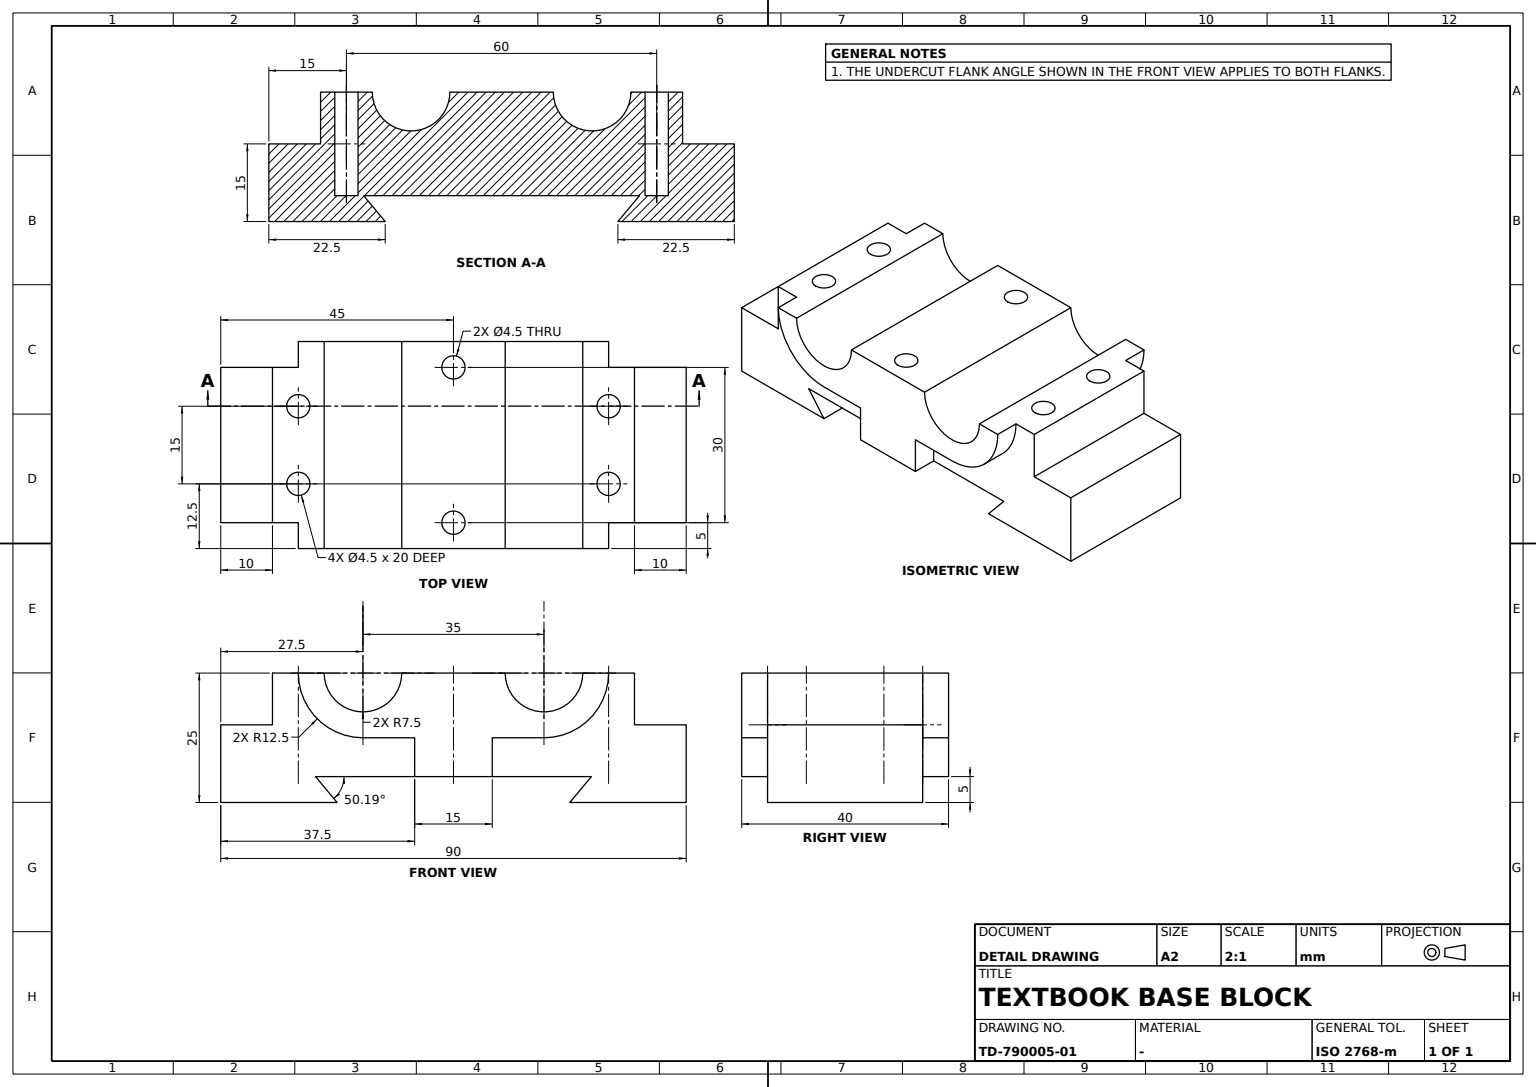
ISO-10303-21;
HEADER;
FILE_DESCRIPTION((''),'2;1');
FILE_NAME('','',(''),(''),'','','');
FILE_SCHEMA(('AUTOMOTIVE_DESIGN'));
ENDSEC;
DATA;
#1=APPLICATION_CONTEXT('');
#2=PRODUCT_CONTEXT('',#1,'mechanical');
#3=PRODUCT('','','',(#2));
#4=PRODUCT_DEFINITION_FORMATION('','',#3);
#5=PRODUCT_DEFINITION_CONTEXT('',#1,'design');
#6=PRODUCT_DEFINITION('','',#4,#5);
#7=PRODUCT_DEFINITION_SHAPE('','',#6);
#8=(LENGTH_UNIT()NAMED_UNIT(*)SI_UNIT(.MILLI.,.METRE.));
#9=(NAMED_UNIT(*)PLANE_ANGLE_UNIT()SI_UNIT($,.RADIAN.));
#10=(NAMED_UNIT(*)SI_UNIT($,.STERADIAN.)SOLID_ANGLE_UNIT());
#11=UNCERTAINTY_MEASURE_WITH_UNIT(LENGTH_MEASURE(0.005),#8,'distance_accuracy_value','');
#12=(GEOMETRIC_REPRESENTATION_CONTEXT(3)GLOBAL_UNCERTAINTY_ASSIGNED_CONTEXT((#11))GLOBAL_UNIT_ASSIGNED_CONTEXT((#8,#9,#10))REPRESENTATION_CONTEXT('',''));
#13=CARTESIAN_POINT('',(15.,35.,20.));
#14=VERTEX_POINT('',#13);
#15=CARTESIAN_POINT('',(15.,30.,20.));
#16=VERTEX_POINT('',#15);
#17=CARTESIAN_POINT('',(15.,0.,20.));
#18=DIRECTION('',(0.,-1.,0.));
#19=VECTOR('',#18,1000.);
#20=LINE('',#17,#19);
#21=EDGE_CURVE('',#14,#16,#20,.T.);
#22=ORIENTED_EDGE('',*,*,#21,.F.);
#23=CARTESIAN_POINT('',(-15.,35.,20.));
#24=VERTEX_POINT('',#23);
#25=CARTESIAN_POINT('',(0.,35.,20.));
#26=DIRECTION('',(1.,0.,0.));
#27=VECTOR('',#26,1000.);
#28=LINE('',#25,#27);
#29=EDGE_CURVE('',#24,#14,#28,.T.);
#30=ORIENTED_EDGE('',*,*,#29,.F.);
#31=CARTESIAN_POINT('',(-15.,30.,20.));
#32=VERTEX_POINT('',#31);
#33=CARTESIAN_POINT('',(-15.,0.,20.));
#34=LINE('',#33,#19);
#35=EDGE_CURVE('',#24,#32,#34,.T.);
#36=ORIENTED_EDGE('',*,*,#35,.T.);
#37=CARTESIAN_POINT('',(-20.,30.,20.));
#38=VERTEX_POINT('',#37);
#39=LINE('',#31,#27);
#40=EDGE_CURVE('',#32,#38,#39,.F.);
#41=ORIENTED_EDGE('',*,*,#40,.T.);
#42=CARTESIAN_POINT('',(-20.,25.,20.));
#43=VERTEX_POINT('',#42);
#44=CARTESIAN_POINT('',(-20.,0.,20.));
#45=LINE('',#44,#19);
#46=EDGE_CURVE('',#38,#43,#45,.T.);
#47=ORIENTED_EDGE('',*,*,#46,.T.);
#48=CARTESIAN_POINT('',(20.,25.,20.));
#49=VERTEX_POINT('',#48);
#50=LINE('',#42,#27);
#51=EDGE_CURVE('',#43,#49,#50,.T.);
#52=ORIENTED_EDGE('',*,*,#51,.T.);
#53=CARTESIAN_POINT('',(20.,30.,20.));
#54=VERTEX_POINT('',#53);
#55=CARTESIAN_POINT('',(20.,0.,20.));
#56=LINE('',#55,#19);
#57=EDGE_CURVE('',#54,#49,#56,.T.);
#58=ORIENTED_EDGE('',*,*,#57,.F.);
#59=LINE('',#15,#27);
#60=EDGE_CURVE('',#16,#54,#59,.T.);
#61=ORIENTED_EDGE('',*,*,#60,.F.);
#62=EDGE_LOOP('',(#22,#30,#36,#41,#47,#52,#58,#61));
#63=FACE_BOUND('',#62,.T.);
#64=CARTESIAN_POINT('',(9.75,30.,20.));
#65=VERTEX_POINT('',#64);
#66=CARTESIAN_POINT('',(7.5,30.,20.));
#67=DIRECTION('',(0.,0.,1.));
#68=AXIS2_PLACEMENT_3D('',#66,#67,#26);
#69=CIRCLE('',#68,2.25);
#70=EDGE_CURVE('',#65,#65,#69,.T.);
#71=ORIENTED_EDGE('',*,*,#70,.F.);
#72=EDGE_LOOP('',(#71));
#73=FACE_BOUND('',#72,.T.);
#74=CARTESIAN_POINT('',(-5.25,30.,20.));
#75=VERTEX_POINT('',#74);
#76=CARTESIAN_POINT('',(-7.5,30.,20.));
#77=AXIS2_PLACEMENT_3D('',#76,#67,#26);
#78=CIRCLE('',#77,2.25);
#79=EDGE_CURVE('',#75,#75,#78,.T.);
#80=ORIENTED_EDGE('',*,*,#79,.F.);
#81=EDGE_LOOP('',(#80));
#82=FACE_BOUND('',#81,.T.);
#83=AXIS2_PLACEMENT_3D('',#25,#67,#18);
#84=PLANE('',#83);
#85=ADVANCED_FACE('',(#63,#73,#82),#84,.T.);
#86=CARTESIAN_POINT('',(-9.75,-30.,0.));
#87=VERTEX_POINT('',#86);
#88=CARTESIAN_POINT('',(-7.5,-30.,0.));
#89=DIRECTION('',(0.,0.,-1.));
#90=DIRECTION('',(-1.,0.,0.));
#91=AXIS2_PLACEMENT_3D('',#88,#89,#90);
#92=CIRCLE('',#91,2.25);
#93=EDGE_CURVE('',#87,#87,#92,.F.);
#94=ORIENTED_EDGE('',*,*,#93,.T.);
#95=EDGE_LOOP('',(#94));
#96=FACE_BOUND('',#95,.T.);
#97=CARTESIAN_POINT('',(0.,-26.666667,0.));
#98=DIRECTION('',(0.,1.,0.));
#99=AXIS2_PLACEMENT_3D('',#97,#89,#98);
#100=PLANE('',#99);
#101=ADVANCED_FACE('',(#96),#100,.F.);
#102=CARTESIAN_POINT('',(-15.,-35.,10.));
#103=VERTEX_POINT('',#102);
#104=CARTESIAN_POINT('',(15.,-35.,10.));
#105=VERTEX_POINT('',#104);
#106=CARTESIAN_POINT('',(0.,-35.,10.));
#107=LINE('',#106,#27);
#108=EDGE_CURVE('',#103,#105,#107,.T.);
#109=ORIENTED_EDGE('',*,*,#108,.F.);
#110=CARTESIAN_POINT('',(-15.,-45.,10.));
#111=VERTEX_POINT('',#110);
#112=CARTESIAN_POINT('',(-15.,45.,10.));
#113=VECTOR('',#98,1000.);
#114=LINE('',#112,#113);
#115=EDGE_CURVE('',#111,#103,#114,.T.);
#116=ORIENTED_EDGE('',*,*,#115,.F.);
#117=CARTESIAN_POINT('',(15.,-45.,10.));
#118=VERTEX_POINT('',#117);
#119=CARTESIAN_POINT('',(0.,-45.,10.));
#120=LINE('',#119,#27);
#121=EDGE_CURVE('',#111,#118,#120,.T.);
#122=ORIENTED_EDGE('',*,*,#121,.T.);
#123=CARTESIAN_POINT('',(15.,45.,10.));
#124=LINE('',#123,#113);
#125=EDGE_CURVE('',#118,#105,#124,.T.);
#126=ORIENTED_EDGE('',*,*,#125,.T.);
#127=EDGE_LOOP('',(#109,#116,#122,#126));
#128=FACE_BOUND('',#127,.T.);
#129=CARTESIAN_POINT('',(0.,45.,10.));
#130=AXIS2_PLACEMENT_3D('',#129,#67,#18);
#131=PLANE('',#130);
#132=ADVANCED_FACE('',(#128),#131,.T.);
#133=CARTESIAN_POINT('',(-15.,35.,10.));
#134=VERTEX_POINT('',#133);
#135=CARTESIAN_POINT('',(15.,35.,10.));
#136=VERTEX_POINT('',#135);
#137=CARTESIAN_POINT('',(0.,35.,10.));
#138=LINE('',#137,#27);
#139=EDGE_CURVE('',#134,#136,#138,.T.);
#140=ORIENTED_EDGE('',*,*,#139,.F.);
#141=CARTESIAN_POINT('',(-15.,35.,0.));
#142=VECTOR('',#67,1000.);
#143=LINE('',#141,#142);
#144=EDGE_CURVE('',#134,#24,#143,.T.);
#145=ORIENTED_EDGE('',*,*,#144,.T.);
#146=ORIENTED_EDGE('',*,*,#29,.T.);
#147=CARTESIAN_POINT('',(15.,35.,0.));
#148=LINE('',#147,#142);
#149=EDGE_CURVE('',#136,#14,#148,.T.);
#150=ORIENTED_EDGE('',*,*,#149,.F.);
#151=EDGE_LOOP('',(#140,#145,#146,#150));
#152=FACE_BOUND('',#151,.T.);
#153=AXIS2_PLACEMENT_3D('',#137,#98,#67);
#154=PLANE('',#153);
#155=ADVANCED_FACE('',(#152),#154,.T.);
#156=CARTESIAN_POINT('',(12.75,0.,0.));
#157=VERTEX_POINT('',#156);
#158=CARTESIAN_POINT('',(15.,0.,0.));
#159=AXIS2_PLACEMENT_3D('',#158,#89,#90);
#160=CIRCLE('',#159,2.25);
#161=EDGE_CURVE('',#157,#157,#160,.F.);
#162=ORIENTED_EDGE('',*,*,#161,.F.);
#163=EDGE_LOOP('',(#162));
#164=FACE_BOUND('',#163,.T.);
#165=CARTESIAN_POINT('',(17.25,0.,20.));
#166=VERTEX_POINT('',#165);
#167=AXIS2_PLACEMENT_3D('',#17,#67,#26);
#168=CIRCLE('',#167,2.25);
#169=EDGE_CURVE('',#166,#166,#168,.T.);
#170=ORIENTED_EDGE('',*,*,#169,.T.);
#171=EDGE_LOOP('',(#170));
#172=FACE_BOUND('',#171,.T.);
#173=CARTESIAN_POINT('',(15.,0.,10.66));
#174=AXIS2_PLACEMENT_3D('',#173,#67,#26);
#175=CYLINDRICAL_SURFACE('',#174,2.25);
#176=ADVANCED_FACE('',(#164,#172),#175,.F.);
#177=CARTESIAN_POINT('',(-15.,-17.5,7.5));
#178=VERTEX_POINT('',#177);
#179=CARTESIAN_POINT('',(-15.,-7.5,7.5));
#180=VERTEX_POINT('',#179);
#181=CARTESIAN_POINT('',(-15.,0.,7.5));
#182=LINE('',#181,#113);
#183=EDGE_CURVE('',#178,#180,#182,.T.);
#184=ORIENTED_EDGE('',*,*,#183,.F.);
#185=CARTESIAN_POINT('',(-20.,-17.5,7.5));
#186=VERTEX_POINT('',#185);
#187=CARTESIAN_POINT('',(17.5,-17.5,7.5));
#188=LINE('',#187,#27);
#189=EDGE_CURVE('',#178,#186,#188,.F.);
#190=ORIENTED_EDGE('',*,*,#189,.T.);
#191=CARTESIAN_POINT('',(-20.,-7.5,7.5));
#192=VERTEX_POINT('',#191);
#193=CARTESIAN_POINT('',(-20.,0.,7.5));
#194=LINE('',#193,#113);
#195=EDGE_CURVE('',#186,#192,#194,.T.);
#196=ORIENTED_EDGE('',*,*,#195,.T.);
#197=CARTESIAN_POINT('',(15.,-7.5,7.5));
#198=VECTOR('',#90,1000.);
#199=LINE('',#197,#198);
#200=EDGE_CURVE('',#180,#192,#199,.T.);
#201=ORIENTED_EDGE('',*,*,#200,.F.);
#202=EDGE_LOOP('',(#184,#190,#196,#201));
#203=FACE_BOUND('',#202,.T.);
#204=CARTESIAN_POINT('',(15.,-17.5,7.5));
#205=AXIS2_PLACEMENT_3D('',#204,#89,#98);
#206=PLANE('',#205);
#207=ADVANCED_FACE('',(#203),#206,.T.);
#208=CARTESIAN_POINT('',(15.,-45.,-5.));
#209=VERTEX_POINT('',#208);
#210=CARTESIAN_POINT('',(15.,-45.,0.));
#211=LINE('',#210,#142);
#212=EDGE_CURVE('',#209,#118,#211,.T.);
#213=ORIENTED_EDGE('',*,*,#212,.T.);
#214=ORIENTED_EDGE('',*,*,#121,.F.);
#215=CARTESIAN_POINT('',(-15.,-45.,-5.));
#216=VERTEX_POINT('',#215);
#217=CARTESIAN_POINT('',(-15.,-45.,0.));
#218=LINE('',#217,#142);
#219=EDGE_CURVE('',#216,#111,#218,.T.);
#220=ORIENTED_EDGE('',*,*,#219,.F.);
#221=CARTESIAN_POINT('',(0.,-45.,-5.));
#222=LINE('',#221,#27);
#223=EDGE_CURVE('',#216,#209,#222,.T.);
#224=ORIENTED_EDGE('',*,*,#223,.T.);
#225=EDGE_LOOP('',(#213,#214,#220,#224));
#226=FACE_BOUND('',#225,.T.);
#227=AXIS2_PLACEMENT_3D('',#221,#98,#67);
#228=PLANE('',#227);
#229=ADVANCED_FACE('',(#226),#228,.F.);
#230=CARTESIAN_POINT('',(15.,45.,-5.));
#231=VERTEX_POINT('',#230);
#232=VERTEX_POINT('',#123);
#233=CARTESIAN_POINT('',(15.,45.,0.));
#234=LINE('',#233,#142);
#235=EDGE_CURVE('',#231,#232,#234,.T.);
#236=ORIENTED_EDGE('',*,*,#235,.F.);
#237=CARTESIAN_POINT('',(-15.,45.,-5.));
#238=VERTEX_POINT('',#237);
#239=CARTESIAN_POINT('',(0.,45.,-5.));
#240=LINE('',#239,#27);
#241=EDGE_CURVE('',#238,#231,#240,.T.);
#242=ORIENTED_EDGE('',*,*,#241,.F.);
#243=VERTEX_POINT('',#112);
#244=CARTESIAN_POINT('',(-15.,45.,0.));
#245=LINE('',#244,#142);
#246=EDGE_CURVE('',#238,#243,#245,.T.);
#247=ORIENTED_EDGE('',*,*,#246,.T.);
#248=LINE('',#129,#27);
#249=EDGE_CURVE('',#243,#232,#248,.T.);
#250=ORIENTED_EDGE('',*,*,#249,.T.);
#251=EDGE_LOOP('',(#236,#242,#247,#250));
#252=FACE_BOUND('',#251,.T.);
#253=AXIS2_PLACEMENT_3D('',#239,#98,#67);
#254=PLANE('',#253);
#255=ADVANCED_FACE('',(#252),#254,.T.);
#256=CARTESIAN_POINT('',(-20.,-7.5,0.));
#257=VERTEX_POINT('',#256);
#258=CARTESIAN_POINT('',(-20.,7.5,0.));
#259=VERTEX_POINT('',#258);
#260=CARTESIAN_POINT('',(-20.,0.,0.));
#261=LINE('',#260,#113);
#262=EDGE_CURVE('',#257,#259,#261,.T.);
#263=ORIENTED_EDGE('',*,*,#262,.F.);
#264=VECTOR('',#89,1000.);
#265=LINE('',#256,#264);
#266=EDGE_CURVE('',#192,#257,#265,.T.);
#267=ORIENTED_EDGE('',*,*,#266,.F.);
#268=ORIENTED_EDGE('',*,*,#195,.F.);
#269=CARTESIAN_POINT('',(-20.,-30.,20.));
#270=VERTEX_POINT('',#269);
#271=CARTESIAN_POINT('',(-20.,-17.5,20.));
#272=AXIS2_PLACEMENT_3D('',#271,#26,#89);
#273=CIRCLE('',#272,12.5);
#274=EDGE_CURVE('',#270,#186,#273,.T.);
#275=ORIENTED_EDGE('',*,*,#274,.F.);
#276=CARTESIAN_POINT('',(-20.,-25.,20.));
#277=VERTEX_POINT('',#276);
#278=CARTESIAN_POINT('',(-20.,35.,20.));
#279=LINE('',#278,#113);
#280=EDGE_CURVE('',#270,#277,#279,.T.);
#281=ORIENTED_EDGE('',*,*,#280,.T.);
#282=CARTESIAN_POINT('',(-20.,-10.,20.));
#283=VERTEX_POINT('',#282);
#284=CIRCLE('',#272,7.5);
#285=EDGE_CURVE('',#277,#283,#284,.T.);
#286=ORIENTED_EDGE('',*,*,#285,.T.);
#287=CARTESIAN_POINT('',(-20.,10.,20.));
#288=VERTEX_POINT('',#287);
#289=EDGE_CURVE('',#288,#283,#45,.T.);
#290=ORIENTED_EDGE('',*,*,#289,.F.);
#291=CARTESIAN_POINT('',(-20.,17.5,20.));
#292=AXIS2_PLACEMENT_3D('',#291,#26,#89);
#293=CIRCLE('',#292,7.5);
#294=EDGE_CURVE('',#288,#43,#293,.T.);
#295=ORIENTED_EDGE('',*,*,#294,.T.);
#296=ORIENTED_EDGE('',*,*,#46,.F.);
#297=CARTESIAN_POINT('',(-20.,17.5,7.5));
#298=VERTEX_POINT('',#297);
#299=CIRCLE('',#292,12.5);
#300=EDGE_CURVE('',#298,#38,#299,.T.);
#301=ORIENTED_EDGE('',*,*,#300,.F.);
#302=CARTESIAN_POINT('',(-20.,7.5,7.5));
#303=VERTEX_POINT('',#302);
#304=LINE('',#185,#19);
#305=EDGE_CURVE('',#298,#303,#304,.T.);
#306=ORIENTED_EDGE('',*,*,#305,.T.);
#307=LINE('',#258,#264);
#308=EDGE_CURVE('',#303,#259,#307,.T.);
#309=ORIENTED_EDGE('',*,*,#308,.T.);
#310=EDGE_LOOP('',(#263,#267,#268,#275,#281,#286,#290,#295,#296,#301,#306,#309));
#311=FACE_BOUND('',#310,.T.);
#312=AXIS2_PLACEMENT_3D('',#260,#26,#98);
#313=PLANE('',#312);
#314=ADVANCED_FACE('',(#311),#313,.F.);
#315=CARTESIAN_POINT('',(5.25,-30.,0.));
#316=VERTEX_POINT('',#315);
#317=CARTESIAN_POINT('',(7.5,-30.,0.));
#318=AXIS2_PLACEMENT_3D('',#317,#89,#90);
#319=CIRCLE('',#318,2.25);
#320=EDGE_CURVE('',#316,#316,#319,.F.);
#321=ORIENTED_EDGE('',*,*,#320,.T.);
#322=EDGE_LOOP('',(#321));
#323=FACE_BOUND('',#322,.T.);
#324=ADVANCED_FACE('',(#323),#100,.F.);
#325=CARTESIAN_POINT('',(-15.,22.5,-5.));
#326=VERTEX_POINT('',#325);
#327=CARTESIAN_POINT('',(15.,22.5,-5.));
#328=VERTEX_POINT('',#327);
#329=CARTESIAN_POINT('',(0.,22.5,-5.));
#330=LINE('',#329,#27);
#331=EDGE_CURVE('',#326,#328,#330,.T.);
#332=ORIENTED_EDGE('',*,*,#331,.T.);
#333=CARTESIAN_POINT('',(15.,26.666667,0.));
#334=VERTEX_POINT('',#333);
#335=CARTESIAN_POINT('',(15.,15.737705,-13.114754));
#336=DIRECTION('',(0.,0.6401844,0.76822128));
#337=VECTOR('',#336,1000.);
#338=LINE('',#335,#337);
#339=EDGE_CURVE('',#328,#334,#338,.T.);
#340=ORIENTED_EDGE('',*,*,#339,.T.);
#341=CARTESIAN_POINT('',(-15.,26.666667,0.));
#342=VERTEX_POINT('',#341);
#343=CARTESIAN_POINT('',(0.,26.666667,0.));
#344=LINE('',#343,#27);
#345=EDGE_CURVE('',#342,#334,#344,.T.);
#346=ORIENTED_EDGE('',*,*,#345,.F.);
#347=CARTESIAN_POINT('',(-15.,15.737705,-13.114754));
#348=LINE('',#347,#337);
#349=EDGE_CURVE('',#326,#342,#348,.T.);
#350=ORIENTED_EDGE('',*,*,#349,.F.);
#351=EDGE_LOOP('',(#332,#340,#346,#350));
#352=FACE_BOUND('',#351,.T.);
#353=DIRECTION('',(0.,0.76822128,-0.6401844));
#354=AXIS2_PLACEMENT_3D('',#329,#353,#336);
#355=PLANE('',#354);
#356=ADVANCED_FACE('',(#352),#355,.F.);
#357=CARTESIAN_POINT('',(5.25,30.,0.));
#358=VERTEX_POINT('',#357);
#359=CARTESIAN_POINT('',(7.5,30.,0.));
#360=AXIS2_PLACEMENT_3D('',#359,#89,#90);
#361=CIRCLE('',#360,2.25);
#362=EDGE_CURVE('',#358,#358,#361,.F.);
#363=ORIENTED_EDGE('',*,*,#362,.T.);
#364=EDGE_LOOP('',(#363));
#365=FACE_BOUND('',#364,.T.);
#366=ADVANCED_FACE('',(#365),#100,.F.);
#367=ORIENTED_EDGE('',*,*,#223,.F.);
#368=CARTESIAN_POINT('',(-15.,-22.5,-5.));
#369=VERTEX_POINT('',#368);
#370=CARTESIAN_POINT('',(-15.,0.,-5.));
#371=LINE('',#370,#113);
#372=EDGE_CURVE('',#216,#369,#371,.T.);
#373=ORIENTED_EDGE('',*,*,#372,.T.);
#374=CARTESIAN_POINT('',(15.,-22.5,-5.));
#375=VERTEX_POINT('',#374);
#376=CARTESIAN_POINT('',(0.,-22.5,-5.));
#377=LINE('',#376,#27);
#378=EDGE_CURVE('',#369,#375,#377,.T.);
#379=ORIENTED_EDGE('',*,*,#378,.T.);
#380=CARTESIAN_POINT('',(15.,0.,-5.));
#381=LINE('',#380,#113);
#382=EDGE_CURVE('',#209,#375,#381,.T.);
#383=ORIENTED_EDGE('',*,*,#382,.F.);
#384=EDGE_LOOP('',(#367,#373,#379,#383));
#385=FACE_BOUND('',#384,.T.);
#386=AXIS2_PLACEMENT_3D('',#221,#89,#98);
#387=PLANE('',#386);
#388=ADVANCED_FACE('',(#385),#387,.T.);
#389=CARTESIAN_POINT('',(9.75,-30.,20.));
#390=VERTEX_POINT('',#389);
#391=CARTESIAN_POINT('',(7.5,-30.,20.));
#392=AXIS2_PLACEMENT_3D('',#391,#67,#26);
#393=CIRCLE('',#392,2.25);
#394=EDGE_CURVE('',#390,#390,#393,.T.);
#395=ORIENTED_EDGE('',*,*,#394,.T.);
#396=EDGE_LOOP('',(#395));
#397=FACE_BOUND('',#396,.T.);
#398=ORIENTED_EDGE('',*,*,#320,.F.);
#399=EDGE_LOOP('',(#398));
#400=FACE_BOUND('',#399,.T.);
#401=CARTESIAN_POINT('',(7.5,-30.,10.66));
#402=AXIS2_PLACEMENT_3D('',#401,#67,#26);
#403=CYLINDRICAL_SURFACE('',#402,2.25);
#404=ADVANCED_FACE('',(#397,#400),#403,.F.);
#405=ORIENTED_EDGE('',*,*,#382,.T.);
#406=CARTESIAN_POINT('',(15.,-26.666667,0.));
#407=VERTEX_POINT('',#406);
#408=CARTESIAN_POINT('',(15.,-15.737705,-13.114754));
#409=DIRECTION('',(0.,-0.6401844,0.76822128));
#410=VECTOR('',#409,1000.);
#411=LINE('',#408,#410);
#412=EDGE_CURVE('',#375,#407,#411,.T.);
#413=ORIENTED_EDGE('',*,*,#412,.T.);
#414=CARTESIAN_POINT('',(15.,-7.5,0.));
#415=VERTEX_POINT('',#414);
#416=LINE('',#158,#113);
#417=EDGE_CURVE('',#407,#415,#416,.T.);
#418=ORIENTED_EDGE('',*,*,#417,.T.);
#419=VERTEX_POINT('',#197);
#420=LINE('',#414,#264);
#421=EDGE_CURVE('',#419,#415,#420,.T.);
#422=ORIENTED_EDGE('',*,*,#421,.F.);
#423=VERTEX_POINT('',#204);
#424=CARTESIAN_POINT('',(15.,0.,7.5));
#425=LINE('',#424,#113);
#426=EDGE_CURVE('',#423,#419,#425,.T.);
#427=ORIENTED_EDGE('',*,*,#426,.F.);
#428=CARTESIAN_POINT('',(15.,-30.,20.));
#429=VERTEX_POINT('',#428);
#430=CARTESIAN_POINT('',(15.,-17.5,20.));
#431=AXIS2_PLACEMENT_3D('',#430,#26,#89);
#432=CIRCLE('',#431,12.5);
#433=EDGE_CURVE('',#429,#423,#432,.T.);
#434=ORIENTED_EDGE('',*,*,#433,.F.);
#435=CARTESIAN_POINT('',(15.,-35.,20.));
#436=VERTEX_POINT('',#435);
#437=LINE('',#13,#113);
#438=EDGE_CURVE('',#436,#429,#437,.T.);
#439=ORIENTED_EDGE('',*,*,#438,.F.);
#440=CARTESIAN_POINT('',(15.,-35.,0.));
#441=LINE('',#440,#142);
#442=EDGE_CURVE('',#105,#436,#441,.T.);
#443=ORIENTED_EDGE('',*,*,#442,.F.);
#444=ORIENTED_EDGE('',*,*,#125,.F.);
#445=ORIENTED_EDGE('',*,*,#212,.F.);
#446=EDGE_LOOP('',(#405,#413,#418,#422,#427,#434,#439,#443,#444,#445));
#447=FACE_BOUND('',#446,.T.);
#448=AXIS2_PLACEMENT_3D('',#158,#26,#98);
#449=PLANE('',#448);
#450=ADVANCED_FACE('',(#447),#449,.T.);
#451=ORIENTED_EDGE('',*,*,#339,.F.);
#452=LINE('',#208,#19);
#453=EDGE_CURVE('',#231,#328,#452,.T.);
#454=ORIENTED_EDGE('',*,*,#453,.F.);
#455=ORIENTED_EDGE('',*,*,#235,.T.);
#456=CARTESIAN_POINT('',(15.,0.,10.));
#457=LINE('',#456,#19);
#458=EDGE_CURVE('',#232,#136,#457,.T.);
#459=ORIENTED_EDGE('',*,*,#458,.T.);
#460=ORIENTED_EDGE('',*,*,#149,.T.);
#461=ORIENTED_EDGE('',*,*,#21,.T.);
#462=CARTESIAN_POINT('',(15.,17.5,7.5));
#463=VERTEX_POINT('',#462);
#464=CARTESIAN_POINT('',(15.,17.5,20.));
#465=AXIS2_PLACEMENT_3D('',#464,#26,#89);
#466=CIRCLE('',#465,12.5);
#467=EDGE_CURVE('',#463,#16,#466,.T.);
#468=ORIENTED_EDGE('',*,*,#467,.F.);
#469=CARTESIAN_POINT('',(15.,7.5,7.5));
#470=VERTEX_POINT('',#469);
#471=LINE('',#204,#19);
#472=EDGE_CURVE('',#463,#470,#471,.T.);
#473=ORIENTED_EDGE('',*,*,#472,.T.);
#474=CARTESIAN_POINT('',(15.,7.5,0.));
#475=VERTEX_POINT('',#474);
#476=LINE('',#474,#264);
#477=EDGE_CURVE('',#470,#475,#476,.T.);
#478=ORIENTED_EDGE('',*,*,#477,.T.);
#479=EDGE_CURVE('',#475,#334,#416,.T.);
#480=ORIENTED_EDGE('',*,*,#479,.T.);
#481=EDGE_LOOP('',(#451,#454,#455,#459,#460,#461,#468,#473,#478,#480));
#482=FACE_BOUND('',#481,.T.);
#483=ADVANCED_FACE('',(#482),#449,.T.);
#484=ORIENTED_EDGE('',*,*,#274,.T.);
#485=ORIENTED_EDGE('',*,*,#189,.F.);
#486=CARTESIAN_POINT('',(-15.,-30.,20.));
#487=VERTEX_POINT('',#486);
#488=CARTESIAN_POINT('',(-15.,-17.5,20.));
#489=AXIS2_PLACEMENT_3D('',#488,#26,#89);
#490=CIRCLE('',#489,12.5);
#491=EDGE_CURVE('',#487,#178,#490,.T.);
#492=ORIENTED_EDGE('',*,*,#491,.F.);
#493=LINE('',#486,#27);
#494=EDGE_CURVE('',#487,#270,#493,.F.);
#495=ORIENTED_EDGE('',*,*,#494,.T.);
#496=EDGE_LOOP('',(#484,#485,#492,#495));
#497=FACE_BOUND('',#496,.T.);
#498=CARTESIAN_POINT('',(17.5,-17.5,20.));
#499=AXIS2_PLACEMENT_3D('',#498,#26,#98);
#500=CYLINDRICAL_SURFACE('',#499,12.5);
#501=ADVANCED_FACE('',(#497),#500,.T.);
#502=ORIENTED_EDGE('',*,*,#169,.F.);
#503=EDGE_LOOP('',(#502));
#504=FACE_BOUND('',#503,.T.);
#505=CARTESIAN_POINT('',(20.,-10.,20.));
#506=VERTEX_POINT('',#505);
#507=LINE('',#282,#27);
#508=EDGE_CURVE('',#283,#506,#507,.T.);
#509=ORIENTED_EDGE('',*,*,#508,.T.);
#510=CARTESIAN_POINT('',(20.,10.,20.));
#511=VERTEX_POINT('',#510);
#512=EDGE_CURVE('',#511,#506,#56,.T.);
#513=ORIENTED_EDGE('',*,*,#512,.F.);
#514=LINE('',#287,#27);
#515=EDGE_CURVE('',#288,#511,#514,.T.);
#516=ORIENTED_EDGE('',*,*,#515,.F.);
#517=ORIENTED_EDGE('',*,*,#289,.T.);
#518=EDGE_LOOP('',(#509,#513,#516,#517));
#519=FACE_BOUND('',#518,.T.);
#520=CARTESIAN_POINT('',(-12.75,0.,20.));
#521=VERTEX_POINT('',#520);
#522=AXIS2_PLACEMENT_3D('',#33,#67,#26);
#523=CIRCLE('',#522,2.25);
#524=EDGE_CURVE('',#521,#521,#523,.T.);
#525=ORIENTED_EDGE('',*,*,#524,.F.);
#526=EDGE_LOOP('',(#525));
#527=FACE_BOUND('',#526,.T.);
#528=ADVANCED_FACE('',(#504,#519,#527),#84,.T.);
#529=CARTESIAN_POINT('',(-5.25,-30.,20.));
#530=VERTEX_POINT('',#529);
#531=CARTESIAN_POINT('',(-7.5,-30.,20.));
#532=AXIS2_PLACEMENT_3D('',#531,#67,#26);
#533=CIRCLE('',#532,2.25);
#534=EDGE_CURVE('',#530,#530,#533,.T.);
#535=ORIENTED_EDGE('',*,*,#534,.F.);
#536=EDGE_LOOP('',(#535));
#537=FACE_BOUND('',#536,.T.);
#538=ORIENTED_EDGE('',*,*,#394,.F.);
#539=EDGE_LOOP('',(#538));
#540=FACE_BOUND('',#539,.T.);
#541=CARTESIAN_POINT('',(-15.,-35.,20.));
#542=VERTEX_POINT('',#541);
#543=LINE('',#23,#113);
#544=EDGE_CURVE('',#542,#487,#543,.T.);
#545=ORIENTED_EDGE('',*,*,#544,.F.);
#546=CARTESIAN_POINT('',(0.,-35.,20.));
#547=LINE('',#546,#27);
#548=EDGE_CURVE('',#542,#436,#547,.T.);
#549=ORIENTED_EDGE('',*,*,#548,.T.);
#550=ORIENTED_EDGE('',*,*,#438,.T.);
#551=CARTESIAN_POINT('',(20.,-30.,20.));
#552=VERTEX_POINT('',#551);
#553=LINE('',#428,#27);
#554=EDGE_CURVE('',#429,#552,#553,.T.);
#555=ORIENTED_EDGE('',*,*,#554,.T.);
#556=CARTESIAN_POINT('',(20.,-25.,20.));
#557=VERTEX_POINT('',#556);
#558=CARTESIAN_POINT('',(20.,35.,20.));
#559=LINE('',#558,#113);
#560=EDGE_CURVE('',#552,#557,#559,.T.);
#561=ORIENTED_EDGE('',*,*,#560,.T.);
#562=LINE('',#276,#27);
#563=EDGE_CURVE('',#277,#557,#562,.T.);
#564=ORIENTED_EDGE('',*,*,#563,.F.);
#565=ORIENTED_EDGE('',*,*,#280,.F.);
#566=ORIENTED_EDGE('',*,*,#494,.F.);
#567=EDGE_LOOP('',(#545,#549,#550,#555,#561,#564,#565,#566));
#568=FACE_BOUND('',#567,.T.);
#569=ADVANCED_FACE('',(#537,#540,#568),#84,.T.);
#570=CARTESIAN_POINT('',(-15.,17.5,7.5));
#571=VERTEX_POINT('',#570);
#572=CARTESIAN_POINT('',(-15.,17.5,20.));
#573=AXIS2_PLACEMENT_3D('',#572,#26,#89);
#574=CIRCLE('',#573,12.5);
#575=EDGE_CURVE('',#571,#32,#574,.T.);
#576=ORIENTED_EDGE('',*,*,#575,.F.);
#577=CARTESIAN_POINT('',(17.5,17.5,7.5));
#578=LINE('',#577,#27);
#579=EDGE_CURVE('',#571,#298,#578,.F.);
#580=ORIENTED_EDGE('',*,*,#579,.T.);
#581=ORIENTED_EDGE('',*,*,#300,.T.);
#582=ORIENTED_EDGE('',*,*,#40,.F.);
#583=EDGE_LOOP('',(#576,#580,#581,#582));
#584=FACE_BOUND('',#583,.T.);
#585=CARTESIAN_POINT('',(17.5,17.5,20.));
#586=AXIS2_PLACEMENT_3D('',#585,#26,#98);
#587=CYLINDRICAL_SURFACE('',#586,12.5);
#588=ADVANCED_FACE('',(#584),#587,.T.);
#589=ORIENTED_EDGE('',*,*,#241,.T.);
#590=ORIENTED_EDGE('',*,*,#453,.T.);
#591=ORIENTED_EDGE('',*,*,#331,.F.);
#592=LINE('',#215,#19);
#593=EDGE_CURVE('',#238,#326,#592,.T.);
#594=ORIENTED_EDGE('',*,*,#593,.F.);
#595=EDGE_LOOP('',(#589,#590,#591,#594));
#596=FACE_BOUND('',#595,.T.);
#597=ADVANCED_FACE('',(#596),#387,.T.);
#598=CARTESIAN_POINT('',(20.,7.5,7.5));
#599=VERTEX_POINT('',#598);
#600=LINE('',#469,#27);
#601=EDGE_CURVE('',#470,#599,#600,.T.);
#602=ORIENTED_EDGE('',*,*,#601,.F.);
#603=ORIENTED_EDGE('',*,*,#472,.F.);
#604=CARTESIAN_POINT('',(20.,17.5,7.5));
#605=VERTEX_POINT('',#604);
#606=EDGE_CURVE('',#463,#605,#578,.T.);
#607=ORIENTED_EDGE('',*,*,#606,.T.);
#608=CARTESIAN_POINT('',(20.,-17.5,7.5));
#609=LINE('',#608,#19);
#610=EDGE_CURVE('',#605,#599,#609,.T.);
#611=ORIENTED_EDGE('',*,*,#610,.T.);
#612=EDGE_LOOP('',(#602,#603,#607,#611));
#613=FACE_BOUND('',#612,.T.);
#614=ADVANCED_FACE('',(#613),#206,.T.);
#615=ORIENTED_EDGE('',*,*,#308,.F.);
#616=CARTESIAN_POINT('',(-15.,7.5,7.5));
#617=VERTEX_POINT('',#616);
#618=LINE('',#469,#198);
#619=EDGE_CURVE('',#617,#303,#618,.T.);
#620=ORIENTED_EDGE('',*,*,#619,.F.);
#621=CARTESIAN_POINT('',(-15.,7.5,0.));
#622=VERTEX_POINT('',#621);
#623=LINE('',#621,#264);
#624=EDGE_CURVE('',#617,#622,#623,.T.);
#625=ORIENTED_EDGE('',*,*,#624,.T.);
#626=CARTESIAN_POINT('',(0.,7.5,0.));
#627=LINE('',#626,#198);
#628=EDGE_CURVE('',#622,#259,#627,.T.);
#629=ORIENTED_EDGE('',*,*,#628,.T.);
#630=EDGE_LOOP('',(#615,#620,#625,#629));
#631=FACE_BOUND('',#630,.T.);
#632=AXIS2_PLACEMENT_3D('',#469,#18,#89);
#633=PLANE('',#632);
#634=ADVANCED_FACE('',(#631),#633,.F.);
#635=ORIENTED_EDGE('',*,*,#285,.F.);
#636=ORIENTED_EDGE('',*,*,#563,.T.);
#637=CARTESIAN_POINT('',(20.,-17.5,20.));
#638=AXIS2_PLACEMENT_3D('',#637,#26,#89);
#639=CIRCLE('',#638,7.5);
#640=EDGE_CURVE('',#557,#506,#639,.T.);
#641=ORIENTED_EDGE('',*,*,#640,.T.);
#642=ORIENTED_EDGE('',*,*,#508,.F.);
#643=EDGE_LOOP('',(#635,#636,#641,#642));
#644=FACE_BOUND('',#643,.T.);
#645=CARTESIAN_POINT('',(0.,-17.5,20.));
#646=AXIS2_PLACEMENT_3D('',#645,#26,#98);
#647=CYLINDRICAL_SURFACE('',#646,7.5);
#648=ADVANCED_FACE('',(#644),#647,.F.);
#649=CARTESIAN_POINT('',(-15.,0.,10.));
#650=LINE('',#649,#19);
#651=EDGE_CURVE('',#243,#134,#650,.T.);
#652=ORIENTED_EDGE('',*,*,#651,.F.);
#653=ORIENTED_EDGE('',*,*,#246,.F.);
#654=ORIENTED_EDGE('',*,*,#593,.T.);
#655=ORIENTED_EDGE('',*,*,#349,.T.);
#656=CARTESIAN_POINT('',(-15.,0.,0.));
#657=LINE('',#656,#113);
#658=EDGE_CURVE('',#622,#342,#657,.T.);
#659=ORIENTED_EDGE('',*,*,#658,.F.);
#660=ORIENTED_EDGE('',*,*,#624,.F.);
#661=LINE('',#177,#19);
#662=EDGE_CURVE('',#571,#617,#661,.T.);
#663=ORIENTED_EDGE('',*,*,#662,.F.);
#664=ORIENTED_EDGE('',*,*,#575,.T.);
#665=ORIENTED_EDGE('',*,*,#35,.F.);
#666=ORIENTED_EDGE('',*,*,#144,.F.);
#667=EDGE_LOOP('',(#652,#653,#654,#655,#659,#660,#663,#664,#665,#666));
#668=FACE_BOUND('',#667,.T.);
#669=AXIS2_PLACEMENT_3D('',#656,#26,#98);
#670=PLANE('',#669);
#671=ADVANCED_FACE('',(#668),#670,.F.);
#672=VERTEX_POINT('',#608);
#673=CIRCLE('',#638,12.5);
#674=EDGE_CURVE('',#552,#672,#673,.T.);
#675=ORIENTED_EDGE('',*,*,#674,.F.);
#676=ORIENTED_EDGE('',*,*,#554,.F.);
#677=ORIENTED_EDGE('',*,*,#433,.T.);
#678=EDGE_CURVE('',#423,#672,#188,.T.);
#679=ORIENTED_EDGE('',*,*,#678,.T.);
#680=EDGE_LOOP('',(#675,#676,#677,#679));
#681=FACE_BOUND('',#680,.T.);
#682=ADVANCED_FACE('',(#681),#500,.T.);
#683=ORIENTED_EDGE('',*,*,#601,.T.);
#684=CARTESIAN_POINT('',(20.,7.5,0.));
#685=VERTEX_POINT('',#684);
#686=LINE('',#684,#264);
#687=EDGE_CURVE('',#599,#685,#686,.T.);
#688=ORIENTED_EDGE('',*,*,#687,.T.);
#689=LINE('',#474,#27);
#690=EDGE_CURVE('',#475,#685,#689,.T.);
#691=ORIENTED_EDGE('',*,*,#690,.F.);
#692=ORIENTED_EDGE('',*,*,#477,.F.);
#693=EDGE_LOOP('',(#683,#688,#691,#692));
#694=FACE_BOUND('',#693,.T.);
#695=ADVANCED_FACE('',(#694),#633,.F.);
#696=ORIENTED_EDGE('',*,*,#515,.T.);
#697=CARTESIAN_POINT('',(20.,17.5,20.));
#698=AXIS2_PLACEMENT_3D('',#697,#26,#89);
#699=CIRCLE('',#698,7.5);
#700=EDGE_CURVE('',#511,#49,#699,.T.);
#701=ORIENTED_EDGE('',*,*,#700,.T.);
#702=ORIENTED_EDGE('',*,*,#51,.F.);
#703=ORIENTED_EDGE('',*,*,#294,.F.);
#704=EDGE_LOOP('',(#696,#701,#702,#703));
#705=FACE_BOUND('',#704,.T.);
#706=CARTESIAN_POINT('',(0.,17.5,20.));
#707=AXIS2_PLACEMENT_3D('',#706,#26,#98);
#708=CYLINDRICAL_SURFACE('',#707,7.5);
#709=ADVANCED_FACE('',(#705),#708,.F.);
#710=ORIENTED_EDGE('',*,*,#421,.T.);
#711=CARTESIAN_POINT('',(20.,-7.5,0.));
#712=VERTEX_POINT('',#711);
#713=LINE('',#414,#27);
#714=EDGE_CURVE('',#415,#712,#713,.T.);
#715=ORIENTED_EDGE('',*,*,#714,.T.);
#716=CARTESIAN_POINT('',(20.,-7.5,7.5));
#717=VERTEX_POINT('',#716);
#718=LINE('',#711,#264);
#719=EDGE_CURVE('',#717,#712,#718,.T.);
#720=ORIENTED_EDGE('',*,*,#719,.F.);
#721=LINE('',#197,#27);
#722=EDGE_CURVE('',#419,#717,#721,.T.);
#723=ORIENTED_EDGE('',*,*,#722,.F.);
#724=EDGE_LOOP('',(#710,#715,#720,#723));
#725=FACE_BOUND('',#724,.T.);
#726=AXIS2_PLACEMENT_3D('',#197,#18,#89);
#727=PLANE('',#726);
#728=ADVANCED_FACE('',(#725),#727,.T.);
#729=ORIENTED_EDGE('',*,*,#467,.T.);
#730=ORIENTED_EDGE('',*,*,#60,.T.);
#731=CIRCLE('',#698,12.5);
#732=EDGE_CURVE('',#605,#54,#731,.T.);
#733=ORIENTED_EDGE('',*,*,#732,.F.);
#734=ORIENTED_EDGE('',*,*,#606,.F.);
#735=EDGE_LOOP('',(#729,#730,#733,#734));
#736=FACE_BOUND('',#735,.T.);
#737=ADVANCED_FACE('',(#736),#587,.T.);
#738=CARTESIAN_POINT('',(-9.75,30.,0.));
#739=VERTEX_POINT('',#738);
#740=CARTESIAN_POINT('',(-7.5,30.,0.));
#741=AXIS2_PLACEMENT_3D('',#740,#89,#90);
#742=CIRCLE('',#741,2.25);
#743=EDGE_CURVE('',#739,#739,#742,.F.);
#744=ORIENTED_EDGE('',*,*,#743,.T.);
#745=EDGE_LOOP('',(#744));
#746=FACE_BOUND('',#745,.T.);
#747=ADVANCED_FACE('',(#746),#100,.F.);
#748=ORIENTED_EDGE('',*,*,#524,.T.);
#749=EDGE_LOOP('',(#748));
#750=FACE_BOUND('',#749,.T.);
#751=CARTESIAN_POINT('',(-17.25,0.,0.));
#752=VERTEX_POINT('',#751);
#753=AXIS2_PLACEMENT_3D('',#656,#89,#90);
#754=CIRCLE('',#753,2.25);
#755=EDGE_CURVE('',#752,#752,#754,.F.);
#756=ORIENTED_EDGE('',*,*,#755,.F.);
#757=EDGE_LOOP('',(#756));
#758=FACE_BOUND('',#757,.T.);
#759=CARTESIAN_POINT('',(-15.,0.,10.66));
#760=AXIS2_PLACEMENT_3D('',#759,#67,#26);
#761=CYLINDRICAL_SURFACE('',#760,2.25);
#762=ADVANCED_FACE('',(#750,#758),#761,.F.);
#763=ORIENTED_EDGE('',*,*,#619,.T.);
#764=ORIENTED_EDGE('',*,*,#305,.F.);
#765=ORIENTED_EDGE('',*,*,#579,.F.);
#766=ORIENTED_EDGE('',*,*,#662,.T.);
#767=EDGE_LOOP('',(#763,#764,#765,#766));
#768=FACE_BOUND('',#767,.T.);
#769=ADVANCED_FACE('',(#768),#206,.T.);
#770=ORIENTED_EDGE('',*,*,#442,.T.);
#771=ORIENTED_EDGE('',*,*,#548,.F.);
#772=CARTESIAN_POINT('',(-15.,-35.,0.));
#773=LINE('',#772,#142);
#774=EDGE_CURVE('',#103,#542,#773,.T.);
#775=ORIENTED_EDGE('',*,*,#774,.F.);
#776=ORIENTED_EDGE('',*,*,#108,.T.);
#777=EDGE_LOOP('',(#770,#771,#775,#776));
#778=FACE_BOUND('',#777,.T.);
#779=AXIS2_PLACEMENT_3D('',#106,#98,#67);
#780=PLANE('',#779);
#781=ADVANCED_FACE('',(#778),#780,.F.);
#782=CARTESIAN_POINT('',(-15.,-7.5,0.));
#783=VERTEX_POINT('',#782);
#784=CARTESIAN_POINT('',(0.,-7.5,0.));
#785=LINE('',#784,#198);
#786=EDGE_CURVE('',#783,#257,#785,.T.);
#787=ORIENTED_EDGE('',*,*,#786,.F.);
#788=LINE('',#782,#264);
#789=EDGE_CURVE('',#180,#783,#788,.T.);
#790=ORIENTED_EDGE('',*,*,#789,.F.);
#791=ORIENTED_EDGE('',*,*,#200,.T.);
#792=ORIENTED_EDGE('',*,*,#266,.T.);
#793=EDGE_LOOP('',(#787,#790,#791,#792));
#794=FACE_BOUND('',#793,.T.);
#795=ADVANCED_FACE('',(#794),#727,.T.);
#796=ORIENTED_EDGE('',*,*,#93,.F.);
#797=EDGE_LOOP('',(#796));
#798=FACE_BOUND('',#797,.T.);
#799=ORIENTED_EDGE('',*,*,#534,.T.);
#800=EDGE_LOOP('',(#799));
#801=FACE_BOUND('',#800,.T.);
#802=CARTESIAN_POINT('',(-7.5,-30.,10.66));
#803=AXIS2_PLACEMENT_3D('',#802,#67,#26);
#804=CYLINDRICAL_SURFACE('',#803,2.25);
#805=ADVANCED_FACE('',(#798,#801),#804,.F.);
#806=ORIENTED_EDGE('',*,*,#70,.T.);
#807=EDGE_LOOP('',(#806));
#808=FACE_BOUND('',#807,.T.);
#809=ORIENTED_EDGE('',*,*,#362,.F.);
#810=EDGE_LOOP('',(#809));
#811=FACE_BOUND('',#810,.T.);
#812=CARTESIAN_POINT('',(7.5,30.,10.66));
#813=AXIS2_PLACEMENT_3D('',#812,#67,#26);
#814=CYLINDRICAL_SURFACE('',#813,2.25);
#815=ADVANCED_FACE('',(#808,#811),#814,.F.);
#816=ORIENTED_EDGE('',*,*,#743,.F.);
#817=EDGE_LOOP('',(#816));
#818=FACE_BOUND('',#817,.T.);
#819=ORIENTED_EDGE('',*,*,#79,.T.);
#820=EDGE_LOOP('',(#819));
#821=FACE_BOUND('',#820,.T.);
#822=CARTESIAN_POINT('',(-7.5,30.,10.66));
#823=AXIS2_PLACEMENT_3D('',#822,#67,#26);
#824=CYLINDRICAL_SURFACE('',#823,2.25);
#825=ADVANCED_FACE('',(#818,#821),#824,.F.);
#826=CARTESIAN_POINT('',(20.,0.,7.5));
#827=LINE('',#826,#113);
#828=EDGE_CURVE('',#672,#717,#827,.T.);
#829=ORIENTED_EDGE('',*,*,#828,.F.);
#830=ORIENTED_EDGE('',*,*,#678,.F.);
#831=ORIENTED_EDGE('',*,*,#426,.T.);
#832=ORIENTED_EDGE('',*,*,#722,.T.);
#833=EDGE_LOOP('',(#829,#830,#831,#832));
#834=FACE_BOUND('',#833,.T.);
#835=ADVANCED_FACE('',(#834),#206,.T.);
#836=ORIENTED_EDGE('',*,*,#755,.T.);
#837=EDGE_LOOP('',(#836));
#838=FACE_BOUND('',#837,.T.);
#839=ORIENTED_EDGE('',*,*,#479,.F.);
#840=ORIENTED_EDGE('',*,*,#690,.T.);
#841=CARTESIAN_POINT('',(20.,0.,0.));
#842=LINE('',#841,#113);
#843=EDGE_CURVE('',#712,#685,#842,.T.);
#844=ORIENTED_EDGE('',*,*,#843,.F.);
#845=ORIENTED_EDGE('',*,*,#714,.F.);
#846=ORIENTED_EDGE('',*,*,#417,.F.);
#847=CARTESIAN_POINT('',(-15.,-26.666667,0.));
#848=VERTEX_POINT('',#847);
#849=LINE('',#97,#27);
#850=EDGE_CURVE('',#848,#407,#849,.T.);
#851=ORIENTED_EDGE('',*,*,#850,.F.);
#852=EDGE_CURVE('',#848,#783,#657,.T.);
#853=ORIENTED_EDGE('',*,*,#852,.T.);
#854=ORIENTED_EDGE('',*,*,#786,.T.);
#855=ORIENTED_EDGE('',*,*,#262,.T.);
#856=ORIENTED_EDGE('',*,*,#628,.F.);
#857=ORIENTED_EDGE('',*,*,#658,.T.);
#858=ORIENTED_EDGE('',*,*,#345,.T.);
#859=EDGE_LOOP('',(#839,#840,#844,#845,#846,#851,#853,#854,#855,#856,#857,#858));
#860=FACE_BOUND('',#859,.T.);
#861=ORIENTED_EDGE('',*,*,#161,.T.);
#862=EDGE_LOOP('',(#861));
#863=FACE_BOUND('',#862,.T.);
#864=ADVANCED_FACE('',(#838,#860,#863),#100,.T.);
#865=ORIENTED_EDGE('',*,*,#491,.T.);
#866=ORIENTED_EDGE('',*,*,#183,.T.);
#867=ORIENTED_EDGE('',*,*,#789,.T.);
#868=ORIENTED_EDGE('',*,*,#852,.F.);
#869=CARTESIAN_POINT('',(-15.,-15.737705,-13.114754));
#870=LINE('',#869,#410);
#871=EDGE_CURVE('',#369,#848,#870,.T.);
#872=ORIENTED_EDGE('',*,*,#871,.F.);
#873=ORIENTED_EDGE('',*,*,#372,.F.);
#874=ORIENTED_EDGE('',*,*,#219,.T.);
#875=ORIENTED_EDGE('',*,*,#115,.T.);
#876=ORIENTED_EDGE('',*,*,#774,.T.);
#877=ORIENTED_EDGE('',*,*,#544,.T.);
#878=EDGE_LOOP('',(#865,#866,#867,#868,#872,#873,#874,#875,#876,#877));
#879=FACE_BOUND('',#878,.T.);
#880=ADVANCED_FACE('',(#879),#670,.F.);
#881=ORIENTED_EDGE('',*,*,#139,.T.);
#882=ORIENTED_EDGE('',*,*,#458,.F.);
#883=ORIENTED_EDGE('',*,*,#249,.F.);
#884=ORIENTED_EDGE('',*,*,#651,.T.);
#885=EDGE_LOOP('',(#881,#882,#883,#884));
#886=FACE_BOUND('',#885,.T.);
#887=ADVANCED_FACE('',(#886),#131,.T.);
#888=ORIENTED_EDGE('',*,*,#378,.F.);
#889=ORIENTED_EDGE('',*,*,#871,.T.);
#890=ORIENTED_EDGE('',*,*,#850,.T.);
#891=ORIENTED_EDGE('',*,*,#412,.F.);
#892=EDGE_LOOP('',(#888,#889,#890,#891));
#893=FACE_BOUND('',#892,.T.);
#894=DIRECTION('',(0.,0.76822128,0.6401844));
#895=AXIS2_PLACEMENT_3D('',#376,#894,#409);
#896=PLANE('',#895);
#897=ADVANCED_FACE('',(#893),#896,.T.);
#898=ORIENTED_EDGE('',*,*,#732,.T.);
#899=ORIENTED_EDGE('',*,*,#57,.T.);
#900=ORIENTED_EDGE('',*,*,#700,.F.);
#901=ORIENTED_EDGE('',*,*,#512,.T.);
#902=ORIENTED_EDGE('',*,*,#640,.F.);
#903=ORIENTED_EDGE('',*,*,#560,.F.);
#904=ORIENTED_EDGE('',*,*,#674,.T.);
#905=ORIENTED_EDGE('',*,*,#828,.T.);
#906=ORIENTED_EDGE('',*,*,#719,.T.);
#907=ORIENTED_EDGE('',*,*,#843,.T.);
#908=ORIENTED_EDGE('',*,*,#687,.F.);
#909=ORIENTED_EDGE('',*,*,#610,.F.);
#910=EDGE_LOOP('',(#898,#899,#900,#901,#902,#903,#904,#905,#906,#907,#908,#909));
#911=FACE_BOUND('',#910,.T.);
#912=AXIS2_PLACEMENT_3D('',#841,#26,#98);
#913=PLANE('',#912);
#914=ADVANCED_FACE('',(#911),#913,.T.);
#915=CLOSED_SHELL('',(#85,#101,#132,#155,#176,#207,#229,#255,#314,#324,#356,#366,#388,#404,#450,#483,#501,#528,#569,#588,#597,#614,#634,#648,#671,#682,#695,#709,#728,#737,#747,#762,#769,#781,#795,#805,#815,#825,#835,#864,#880,#887,#897,#914));
#916=MANIFOLD_SOLID_BREP('',#915);
#917=ADVANCED_BREP_SHAPE_REPRESENTATION('',(#916),#12);
#918=SHAPE_DEFINITION_REPRESENTATION(#7,#917);
ENDSEC;
END-ISO-10303-21;
